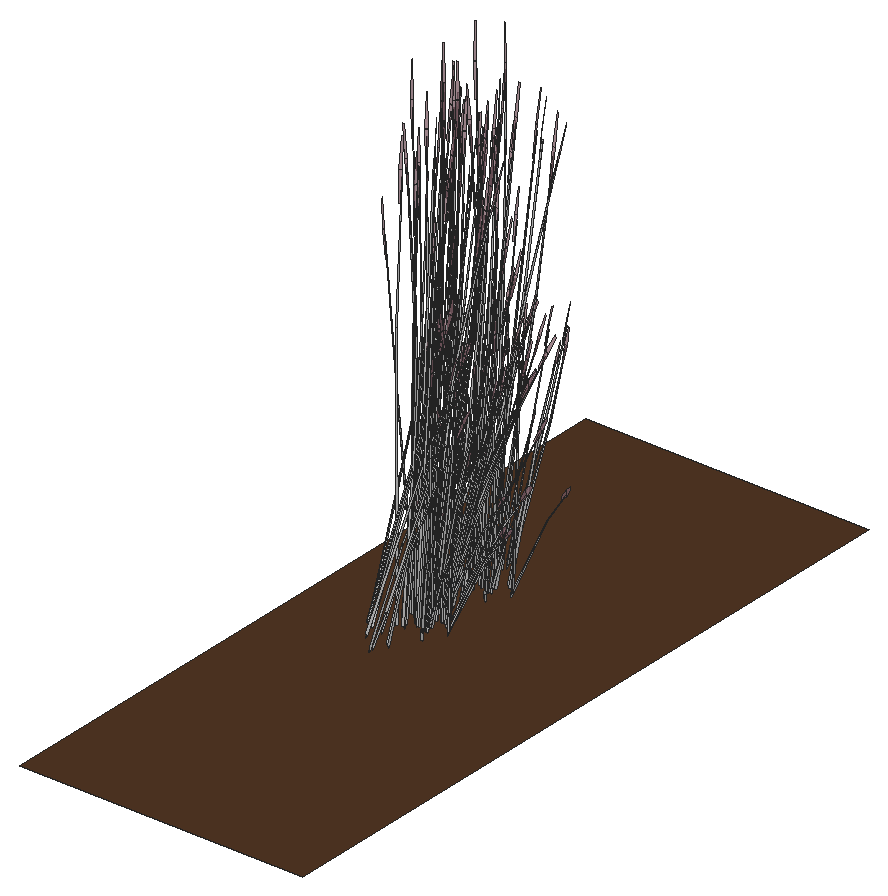
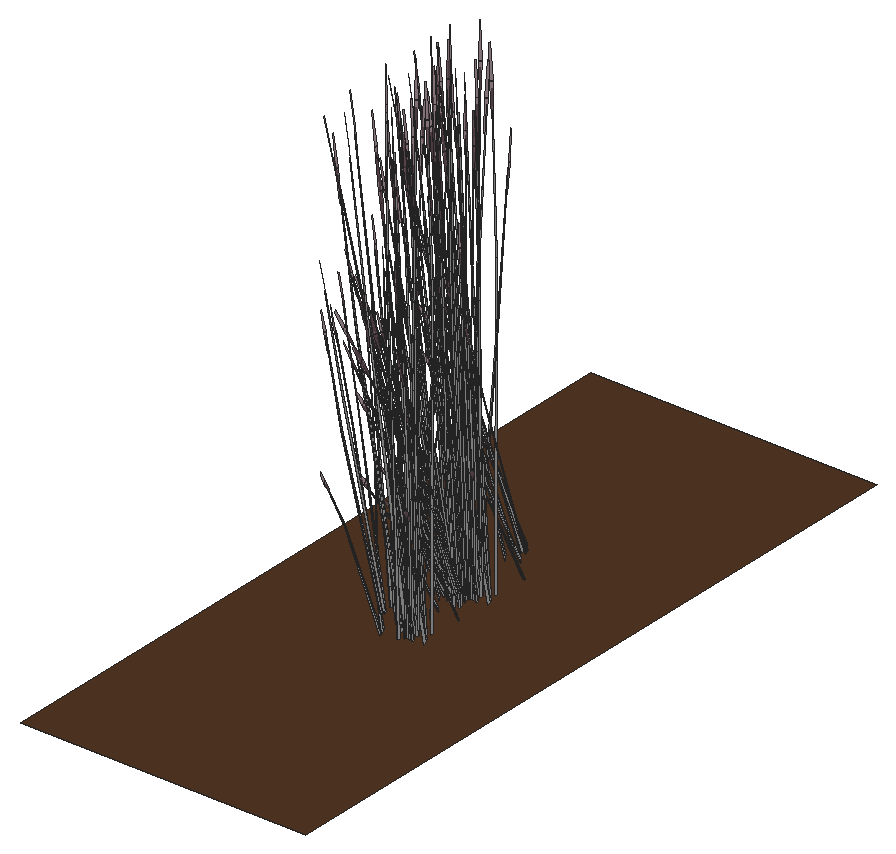
# SketchUp Ruby script. Lengths in inches.
U = 1.inch
M = Sketchup.active_model
def pt(a) = Geom::Point3d.new(a.map { |v| v * U })
def face(e, loops, mat)
  f = e.add_face(loops[0].map { |a| pt(a) })
  loops[1..].each { |l| e.add_face(l.map { |a| pt(a) }).erase! }
  f.material = f.back_material = mat if mat
  f
end
# faces: each face lists its corners as indices into pts; further lists are holes
def faces(e, pts, list, mat = nil) = list.each { |f| face(e, (f[0].is_a?(Array) ? f : [f]).map { |l| l.map { |i| pts[i] } }, mat) }
# xy, xz, yz: faces in a plane at the given z, y or x. An outline is a flat list of corners, or four numbers for a rectangle; further outlines are holes
def ring(l) = l.size == 4 ? [[l[0], l[1]], [l[2], l[1]], [l[2], l[3]], [l[0], l[3]]] : l.each_slice(2).to_a
def flat(e, list, mat, &to3) = list.each { |f| face(e, (f[0].is_a?(Array) ? f : [f]).map { |l| ring(l).map { |u, v| to3.(u, v) } }, mat) }
def xy(e, z, list, mat = nil) = flat(e, list, mat) { |x, y| [x, y, z] }
def xz(e, y, list, mat = nil) = flat(e, list, mat) { |x, z| [x, y, z] }
def yz(e, x, list, mat = nil) = flat(e, list, mat) { |y, z| [x, y, z] }
def lines(e, pts, list) = list.each { |a, b| e.add_line(pt(pts[a]), pt(pts[b])) }
# prism: a flat outline (further loops are holes) pulled along v
def prism(e, loops, v, mat = nil)
  f = face(e, loops, mat); d = Geom::Vector3d.new(v.map { |x| x * U })
  f.pushpull(f.normal.samedirection?(d) ? d.length : -d.length)
end
def box(e, o, s, mat = nil) = prism(e, [[o, [o[0] + s[0], o[1], o[2]], [o[0] + s[0], o[1] + s[1], o[2]], [o[0], o[1] + s[1], o[2]]]], [0, 0, s[2]], mat)
def at(x, y, z, deg = 0) = Geom::Transformation.translation(pt([x, y, z])) * Geom::Transformation.rotation(ORIGIN, Z_AXIS, deg.degrees)
def axes(o, x, y, z) = Geom::Transformation.new([*x, 0, *y, 0, *z, 0, *pt(o).to_a, 1])
def part(name) = M.definitions.add(name)
# library, detail: a bought-in or finely detailed component or shape, given as its bounding box
def library(name, o, s) = part(name).tap { |d| box(d.entities, o, s) }
def detail(e, o, s) = box(e.add_group.entities, o, s)
def put(e, d, t, mat = nil) = e.add_instance(d, t).tap { |i| i.material = mat if mat }
def group(e, t, mat = nil) = e.add_group.tap { |g| g.transformation = t; g.material = mat if mat }.entities
root = M.entities
M.materials.add("LightPink_Translucent").color = [144, 107, 117]
M.materials["LightPink_Translucent"].alpha = 0.75
M.materials.add("Wood_Veneer_15_1K").color = [81, 54, 35]
M.materials.add("[_0053_Ivory_]").color = [200, 200, 200]
c1 = part("blade")
p = [[2.15,0.21,22],[0,0.17,0],[0.09,0.45,0],[2.18,0.31,22],[2.29,0.31,22],[0.38,0.45,0],
  [2.48,0.24,33],[2.49,0.24,33],[2.48,0.22,33]]
faces(c1.entities,p,[[0,1,2,3],[4,5,2,3],[6,3,4,7],[8,0,3,6]])
c2 = part("seeds")
p = [[0.3,-0.1,1.38],[-0.01,-0.03,1.59],[-0.01,-0.03,0.03],[0.14,-0.07,-0.07],[0.29,-0.03,3],[0.15,0.01,3.11]]
faces(c2.entities,p,[[0,1,2,3],[1,0,4,5]],"LightPink_Translucent")
c3 = part("blade with seeds")
put(c3.entities,c1,at(0,0,0))
put(c3.entities,c2,axes([2.4,0.25,30.99],[1.5799,-0.05474,1.17369],[-0.12525,1.92788,0.29478],[-0.07173,-0.02425,1.56792]))
xy(root,252,[[617.51,269.15,653.51,359.15]],"Wood_Veneer_15_1K")
put(root,c3,axes([631.24,314.625,253.86],[0.29468,-0.56664,-0.44739],[0.61229,0.27271,0.21531],[0,-0.13062,1.43643]),"[_0053_Ivory_]")
put(root,c3,axes([631.24,324.73,253.86],[0.29468,-0.56664,-0.44739],[0.61229,0.27271,0.21531],[0,-0.13062,1.43643]),"[_0053_Ivory_]")
put(root,c3,axes([631.99,316.45,253.86],[-0.19817,-0.54216,0],[0.56587,-0.18986,0],[0,0,1.54371]),"[_0053_Ivory_]")
put(root,c3,axes([631.27,307.21,253.15],[0.09829,-0.03422,1.76342],[0.59126,0.18834,-0.26939],[0.01729,0.21228,0.30037]),"[_0053_Ivory_]")
put(root,c3,axes([631.27,317.6,253.15],[0.09829,-0.03422,1.76342],[0.59126,0.18834,-0.26939],[0.01729,0.21228,0.30037]),"[_0053_Ivory_]")
put(root,c3,axes([631.4,307.4,256.18],[-0.1831,0.48359,-0.35414],[-0.53419,-0.14105,0.4572],[0.04898,0.1947,0.87481]),"[_0053_Ivory_]")
put(root,c3,axes([631.4,317.79,256.18],[-0.1831,0.48359,-0.35414],[-0.53419,-0.14105,0.4572],[0.04898,0.1947,0.87481]),"[_0053_Ivory_]")
put(root,c3,axes([632.79,315.38,253.86],[-0.29468,0.56664,-0.44739],[-0.61229,-0.27271,0.21531],[0,0.13062,1.43643]),"[_0053_Ivory_]")
put(root,c3,axes([633.95,315.04,254.13],[-0.47719,-0.45806,0.17642],[0.48088,-0.44429,0.35086],[-0.0527,0.09355,1.60407]),"[_0053_Ivory_]")
put(root,c3,axes([632.31,314.78,253.86],[0,-0.72763,0],[0.75945,0,0],[0,0,1.79456]),"[_0053_Ivory_]")
put(root,c3,axes([632.31,324.88,253.86],[0,-0.72763,0],[0.75945,0,0],[0,0,1.79456]),"[_0053_Ivory_]")
put(root,c3,axes([631.6,314.91,254.09],[0.68433,0.30479,0.24065],[-0.32934,0.63331,0.50002],[0,-0.14599,1.60543]),"[_0053_Ivory_]")
put(root,c3,axes([631.6,325.01,254.09],[0.68433,0.30479,0.24065],[-0.32934,0.63331,0.50002],[0,-0.14599,1.60543]),"[_0053_Ivory_]")
put(root,c3,axes([632.6875,315.07,253.95],[0,0.72727,-0.05637],[-0.75945,0,0],[0,0.02286,1.79368]),"[_0053_Ivory_]")
put(root,c3,axes([631.38,314.48,254.37],[-0.65953,0.03882,0.44739],[-0.05964,-0.64439,-0.21531],[0.11807,-0.06531,1.43643]),"[_0053_Ivory_]")
put(root,c3,axes([631.38,324.59,254.37],[-0.65953,0.03882,0.44739],[-0.05964,-0.64439,-0.21531],[0.11807,-0.06531,1.43643]),"[_0053_Ivory_]")
put(root,c3,axes([631.07,313.375,254.13],[-0.17545,0.62497,0.17642],[-0.64204,-0.17686,0.35086],[0.11091,-0.00304,1.60407]),"[_0053_Ivory_]")
put(root,c3,axes([631.07,323.48,254.13],[-0.17545,0.62497,0.17642],[-0.64204,-0.17686,0.35086],[0.11091,-0.00304,1.60407]),"[_0053_Ivory_]")
put(root,c3,axes([632.32,316.47,253.94],[0.26406,0.72244,-0.06012],[-0.7545,0.25315,0],[0.00922,0.02523,1.72173]),"[_0053_Ivory_]")
put(root,c3,axes([630.76,312.61,254.03],[-0.37973,-0.63014,0],[0.6353,-0.35142,-0.51607],[0.14469,-0.08004,1.63711]),"[_0053_Ivory_]")
put(root,c3,axes([630.76,322.71,254.03],[-0.37973,-0.63014,0],[0.6353,-0.35142,-0.51607],[0.14469,-0.08004,1.63711]),"[_0053_Ivory_]")
put(root,c3,axes([631.46,306.96,256.63],[0.28988,0.51132,-0.71045],[-0.59671,0.28496,0.08574],[0.06778,0.24706,1.00501]),"[_0053_Ivory_]")
put(root,c3,axes([631.46,317.35,256.63],[0.28988,0.51132,-0.71045],[-0.59671,0.28496,0.08574],[0.06778,0.24706,1.00501]),"[_0053_Ivory_]")
put(root,c3,axes([634.51,315.53,253.85],[-0.75908,-0.00503,-0.04976],[0,-0.70283,0.49943],[-0.02386,0.16,1.58352]),"[_0053_Ivory_]")
put(root,c3,axes([633.01,313.41,254.13],[-0.65264,0.16691,0.17642],[-0.16115,-0.62115,0.35086],[0.05821,0.0905,1.60407]),"[_0053_Ivory_]")
put(root,c3,axes([632.35,321.1875,254.42],[0.07791,0.3667,1.1486],[-0.43222,-0.2031,0.84392],[0.04651,-0.18776,0.25299]),"[_0053_Ivory_]")
put(root,c3,axes([631.95,314.32,254.01],[-0.50358,0.57069,0.45755],[-0.59827,-0.50377,0.17955],[0.1214,-0.05695,1.58856]),"[_0053_Ivory_]")
put(root,c3,axes([631.95,324.42,254.01],[-0.50358,0.57069,0.45755],[-0.59827,-0.50377,0.17955],[0.1214,-0.05695,1.58856]),"[_0053_Ivory_]")
put(root,c3,axes([632.81,315.22,253.87],[0.42396,0.40619,0],[-0.42396,0.40619,0],[0,0,1.69266]),"[_0053_Ivory_]")
put(root,c3,axes([632.8,314.74,254.37],[0.29468,-0.56664,0.44739],[0.61229,0.27271,-0.21531],[0,0.13062,1.43643]),"[_0053_Ivory_]")
put(root,c3,axes([632.55,316.71,253.86],[0.61229,0.28233,0],[-0.29468,0.58663,0],[0,0,1.74954]),"[_0053_Ivory_]")
put(root,c3,axes([631.67,307.07,256.33],[0.59704,0.15764,-0.51099],[-0.20464,0.54049,-0.3958],[0.05475,0.21761,0.97773]),"[_0053_Ivory_]")
put(root,c3,axes([631.67,317.46,256.33],[0.59704,0.15764,-0.51099],[-0.20464,0.54049,-0.3958],[0.05475,0.21761,0.97773]),"[_0053_Ivory_]")
put(root,c3,axes([632.6,314.61,254.03],[-0.76764,-0.13249,0.49198],[0.15622,-0.74829,0.19306],[0.11218,0.07226,1.70813]),"[_0053_Ivory_]")
put(root,c3,axes([634.35,315.63,253.68],[-0.42396,0.39235,-0.30978],[-0.42396,-0.39235,0.30978],[0,0.12637,1.38974]),"[_0053_Ivory_]")
put(root,c3,axes([633.14,315.56,253.75],[0.2227,0.57576,-0.69212],[-0.64151,0.20736,-0.18165],[0.02462,0.19497,1.52773]),"[_0053_Ivory_]")
put(root,c3,axes([632.82,314.9375,253.86],[0.67951,0,0],[0,0.65103,0],[0,0,1.78407]),"[_0053_Ivory_]")
put(root,c3,axes([632.82,325.04,253.86],[0.67951,0,0],[0,0.65103,0],[0,0,1.78407]),"[_0053_Ivory_]")
put(root,c3,axes([632.17,314.22,254.37],[-0.36485,-0.52782,0.44739],[0.55265,-0.37168,-0.21531],[0.11807,0.06531,1.43643]),"[_0053_Ivory_]")
put(root,c3,axes([632.17,324.33,254.37],[-0.36485,-0.52782,0.44739],[0.55265,-0.37168,-0.21531],[0.11807,0.06531,1.43643]),"[_0053_Ivory_]")
put(root,c3,axes([631.5,314.35,254.32],[-0.07077,-0.71755,-0.29095],[0.73712,-0.04339,-0.50002],[0.1298,-0.09558,1.59708]),"[_0053_Ivory_]")
put(root,c3,axes([631.5,324.45,254.32],[-0.07077,-0.71755,-0.29095],[0.73712,-0.04339,-0.50002],[0.1298,-0.09558,1.59708]),"[_0053_Ivory_]")
put(root,c3,axes([633.06,314.87,254.27],[0.56587,-0.18339,0.1448],[0.19817,0.52368,-0.41347],[0,0.11525,1.26744]),"[_0053_Ivory_]")
put(root,c3,axes([633.27,322.95,256.33],[-0.43478,-0.42253,-0.51099],[0.45929,-0.37004,-0.3958],[0.06615,-0.21468,0.97773]),"[_0053_Ivory_]")
put(root,c3,axes([632.86,314.91,254.32],[0.68399,0.30005,-0.29095],[-0.32934,0.63331,-0.50002],[0.0215,0.15549,1.59708]),"[_0053_Ivory_]")
put(root,c3,axes([631.41,312.76,253.68],[0.56663,0.1556,-0.30978],[-0.14267,0.54795,0.30978],[0.11423,-0.06319,1.38974]),"[_0053_Ivory_]")
put(root,c3,axes([631.41,322.86,253.68],[0.56663,0.1556,-0.30978],[-0.14267,0.54795,0.30978],[0.11423,-0.06319,1.38974]),"[_0053_Ivory_]")
put(root,c3,axes([632.98,322.2,254.24],[-0.17264,0.12729,1.43002],[-0.51703,-0.22279,-0.30754],[0.09584,-0.27707,0.61141]),"[_0053_Ivory_]")
put(root,c3,axes([634.35,315.06,254.13],[0,-0.62885,0.49651],[0.67951,0,0],[0,0.14322,1.57504]),"[_0053_Ivory_]")
put(root,c3,axes([634.64,315.64,253.67],[0,0.62885,-0.49651],[-0.67951,0,0],[0,0.14322,1.57504]),"[_0053_Ivory_]")
put(root,c3,axes([631.27,312.51,253.67],[0.56842,-0.31443,-0.49651],[0.33976,0.56381,0],[0.12946,-0.07161,1.57504]),"[_0053_Ivory_]")
put(root,c3,axes([631.27,322.61,253.67],[0.56842,-0.31443,-0.49651],[0.33976,0.56381,0],[0.12946,-0.07161,1.57504]),"[_0053_Ivory_]")
put(root,c3,axes([632.01,305.95,255.53],[-0.13883,-0.2019,1.71376],[0.64153,-0.16998,0.13857],[0.14499,0.31697,0.73262]),"[_0053_Ivory_]")
put(root,c3,axes([632.01,316.34,255.53],[-0.13883,-0.2019,1.71376],[0.64153,-0.16998,0.13857],[0.14499,0.31697,0.73262]),"[_0053_Ivory_]")
put(root,c3,axes([632.41,314.07,254.27],[0.11717,-0.56122,0.1448],[0.57245,0.09742,-0.41347],[0.10418,0.05763,1.26744]),"[_0053_Ivory_]")
put(root,c3,axes([632.41,324.18,254.27],[0.11717,-0.56122,0.1448],[0.57245,0.09742,-0.41347],[0.10418,0.05763,1.26744]),"[_0053_Ivory_]")
put(root,c3,axes([633.23,313.09,254.13],[-0.56842,-0.31443,0.49651],[0.33976,-0.56381,0],[0.12946,0.07161,1.57504]),"[_0053_Ivory_]")
put(root,c3,axes([633.23,323.2,254.13],[-0.56842,-0.31443,0.49651],[0.33976,-0.56381,0],[0.12946,0.07161,1.57504]),"[_0053_Ivory_]")
put(root,c3,axes([633.4,323.15,256.63],[0.0158,-0.58168,-0.71045],[0.66548,0.03907,0.08574],[0.07023,-0.24643,1.00501]),"[_0053_Ivory_]")
put(root,c3,axes([632.73,316.38,253.84],[0.63764,-0.21337,-0.19198],[0.22406,0.61462,0.00008],[0.07038,-0.02358,1.73897]),"[_0053_Ivory_]")
put(root,c3,axes([632.74,314.55,253.86],[0.36485,0.52782,-0.44739],[-0.55265,0.37168,0.21531],[0.11807,0.06531,1.43643]),"[_0053_Ivory_]")
put(root,c3,axes([633.68,322.8,256.18],[0.41095,-0.33109,-0.35414],[0.38901,0.37805,0.4572],[0.05919,-0.19208,0.87481]),"[_0053_Ivory_]")
put(root,c3,axes([633.78,316.95,254.42],[-0.34197,-0.18082,1.1486],[0.44156,-0.18372,0.84392],[0.1191,0.15563,0.25299]),"[_0053_Ivory_]")
put(root,c3,axes([632.56,306.36,254.24],[0.01072,-0.20846,1.43002],[0.51218,-0.23285,-0.30754],[0.15811,0.2495,0.61141]),"[_0053_Ivory_]")
put(root,c3,axes([632.56,316.75,254.24],[0.01072,-0.20846,1.43002],[0.51218,-0.23285,-0.30754],[0.15811,0.2495,0.61141]),"[_0053_Ivory_]")
put(root,c3,axes([631.95,313.8,253.71],[0.40909,-0.47266,-0.62353],[0.50819,0.4286,-0.16365],[0.16393,-0.11791,1.37633]),"[_0053_Ivory_]")
put(root,c3,axes([631.95,323.9,253.71],[0.40909,-0.47266,-0.62353],[0.50819,0.4286,-0.16365],[0.16393,-0.11791,1.37633]),"[_0053_Ivory_]")
put(root,c3,axes([633.74,313.38,253.68],[0.14267,0.54795,-0.30978],[-0.56663,0.1556,0.30978],[0.11423,0.06319,1.38974]),"[_0053_Ivory_]")
put(root,c3,axes([634.81,315.16,254.03],[0.75945,0,0],[0,0.70283,-0.51607],[0,0.16007,1.63711]),"[_0053_Ivory_]")
put(root,c3,axes([632.35,314.25,254.32],[0.61322,-0.4175,-0.29095],[0.40778,0.58992,-0.50002],[0.1513,0.05991,1.59708]),"[_0053_Ivory_]")
put(root,c3,axes([632.35,324.36,254.32],[0.61322,-0.4175,-0.29095],[0.40778,0.58992,-0.50002],[0.1513,0.05991,1.59708]),"[_0053_Ivory_]")
put(root,c3,axes([633.83,307.38,254.32],[-0.38947,-0.01972,1.0506],[0.25721,-0.41888,0.58006],[0.15386,0.14882,0.8241]),"[_0053_Ivory_]")
put(root,c3,axes([633.83,317.77,254.32],[-0.38947,-0.01972,1.0506],[0.25721,-0.41888,0.58006],[0.15386,0.14882,0.8241]),"[_0053_Ivory_]")
put(root,c3,axes([632.65,322.85,255.53],[-0.11309,0.21615,1.71376],[-0.47441,-0.44731,0.13857],[0.21402,-0.27879,0.73262]),"[_0053_Ivory_]")
put(root,c3,axes([630.81,313.88,253.25],[-0.59782,0.25177,1.28929],[-0.19028,-0.72239,0.50096],[0.36709,0.01202,1.46642]),"[_0053_Ivory_]")
put(root,c3,axes([630.81,323.99,253.25],[-0.59782,0.25177,1.28929],[-0.19028,-0.72239,0.50096],[0.36709,0.01202,1.46642]),"[_0053_Ivory_]")
put(root,c3,axes([633,306.8,256.33],[0.59932,-0.14948,-0.51099],[0.10484,0.56611,-0.3958],[0.16097,0.16223,0.97773]),"[_0053_Ivory_]")
put(root,c3,axes([633,317.19,256.33],[0.59932,-0.14948,-0.51099],[0.10484,0.56611,-0.3958],[0.16097,0.16223,0.97773]),"[_0053_Ivory_]")
put(root,c3,axes([633.55,312.76,254.03],[0.37973,-0.63014,0],[0.6353,0.35142,-0.51607],[0.14469,0.08004,1.63711]),"[_0053_Ivory_]")
put(root,c3,axes([633.55,322.87,254.03],[0.37973,-0.63014,0],[0.6353,0.35142,-0.51607],[0.14469,0.08004,1.63711]),"[_0053_Ivory_]")
put(root,c3,axes([634.19,312.49,253.15],[-0.0909,-0.04954,1.76342],[-0.2335,-0.55347,-0.26939],[0.15752,-0.1502,0.30037]),"[_0053_Ivory_]")
put(root,c3,axes([634.19,322.6,253.15],[-0.0909,-0.04954,1.76342],[-0.2335,-0.55347,-0.26939],[0.15752,-0.1502,0.30037]),"[_0053_Ivory_]")
put(root,c3,axes([633.9,313.14,253.67],[0.56842,0.31443,-0.49651],[-0.33976,0.56381,0],[0.12946,0.07161,1.57504]),"[_0053_Ivory_]")
put(root,c3,axes([633.9,323.25,253.67],[0.56842,0.31443,-0.49651],[-0.33976,0.56381,0],[0.12946,0.07161,1.57504]),"[_0053_Ivory_]")
put(root,c3,axes([633.87,317.62,253.15],[0.04425,-0.09079,1.76342],[0.55709,-0.26738,-0.26939],[0.16889,0.13839,0.30037]),"[_0053_Ivory_]")
put(root,c3,axes([634.17,313.82,256.33],[-0.15602,-0.5742,-0.51099],[0.59087,-0.10045,-0.3958],[0.16933,-0.15423,0.97773]),"[_0053_Ivory_]")
put(root,c3,axes([634.17,323.92,256.33],[-0.15602,-0.5742,-0.51099],[0.59087,-0.10045,-0.3958],[0.16933,-0.15423,0.97773]),"[_0053_Ivory_]")
put(root,c3,axes([635.21,316.78,255.58],[-0.11624,-0.52862,-0.03492],[0.54943,-0.12153,-0.15832],[0.11473,0.03351,0.52218]),"[_0053_Ivory_]")
put(root,c3,axes([633.07,314.35,253.71],[0.63179,0.1031,-0.62353],[-0.13332,0.63596,-0.16365],[0.18854,0.07706,1.37633]),"[_0053_Ivory_]")
put(root,c3,axes([635.76,314.72,253.91],[-0.37654,-0.40212,-0.06488],[0.4124,-0.36845,-0.29416],[0.11685,-0.02594,0.97024]),"[_0053_Ivory_]")
put(root,c3,axes([635.76,324.83,253.91],[-0.37654,-0.40212,-0.06488],[0.4124,-0.36845,-0.29416],[0.11685,-0.02594,0.97024]),"[_0053_Ivory_]")
put(root,c3,axes([634.9,312.68,254.42],[-0.2023,0.32011,1.1486],[-0.17388,-0.43009,0.84392],[0.16708,-0.10777,0.25299]),"[_0053_Ivory_]")
put(root,c3,axes([634.9,322.78,254.42],[-0.2023,0.32011,1.1486],[-0.17388,-0.43009,0.84392],[0.16708,-0.10777,0.25299]),"[_0053_Ivory_]")
put(root,c3,axes([632.94,315.71,255.53],[-0.2256,-0.10835,1.71376],[0.46687,-0.45453,0.13857],[0.29098,0.20505,0.73262]),"[_0053_Ivory_]")
put(root,c3,axes([634.61,313.88,256.18],[0.52868,-0.08987,-0.35414],[0.1396,0.51376,0.4572],[0.1515,-0.13799,0.87481]),"[_0053_Ivory_]")
put(root,c3,axes([634.61,323.98,256.18],[0.52868,-0.08987,-0.35414],[0.1396,0.51376,0.4572],[0.1515,-0.13799,0.87481]),"[_0053_Ivory_]")
put(root,c3,axes([634.1875,314.05,256.63],[0.31725,-0.49618,-0.71045],[0.55593,0.35263,0.08574],[0.18942,-0.17977,1.00501]),"[_0053_Ivory_]")
put(root,c3,axes([634.1875,324.16,256.63],[0.31725,-0.49618,-0.71045],[0.55593,0.35263,0.08574],[0.18942,-0.17977,1.00501]),"[_0053_Ivory_]")
put(root,c3,axes([634.18,316.72,256.18],[0.34557,0.39372,-0.35414],[-0.39459,0.37271,0.4572],[0.20048,0.05671,0.87481]),"[_0053_Ivory_]")
put(root,c3,axes([634.45,315.09,256.33],[0.16454,-0.57202,-0.51099],[0.56413,0.19607,-0.3958],[0.22713,-0.05245,0.97773]),"[_0053_Ivory_]")
put(root,c3,axes([634.45,325.2,256.33],[0.16454,-0.57202,-0.51099],[0.56413,0.19607,-0.3958],[0.22713,-0.05245,0.97773]),"[_0053_Ivory_]")
put(root,c3,axes([635.86,315.46,254.42],[-0.37526,0.10382,1.1486],[0.17664,-0.42906,0.84392],[0.19907,0.02936,0.25299]),"[_0053_Ivory_]")
put(root,c3,axes([634.65,313.59,254.24],[-0.21697,-0.01863,1.43002],[-0.22228,-0.49966,-0.30754],[0.26655,-0.14135,0.61141]),"[_0053_Ivory_]")
put(root,c3,axes([634.65,323.7,254.24],[-0.21697,-0.01863,1.43002],[-0.22228,-0.49966,-0.30754],[0.26655,-0.14135,0.61141]),"[_0053_Ivory_]")
put(root,c3,axes([634.79,315.35,256.18],[0.50475,0.17543,-0.35414],[-0.14722,0.5118,0.4572],[0.20322,-0.04693,0.87481]),"[_0053_Ivory_]")
put(root,c3,axes([634.79,325.46,256.18],[0.50475,0.17543,-0.35414],[-0.14722,0.5118,0.4572],[0.20322,-0.04693,0.87481]),"[_0053_Ivory_]")
put(root,c3,axes([633.82,316.46,256.63],[0.60713,0.01514,-0.71045],[-0.04078,0.63759,0.08574],[0.25721,0.06729,1.00501]),"[_0053_Ivory_]")
put(root,c3,axes([635.05,315.26,253.64],[-0.39118,0.07547,1.41583],[-0.06226,-0.6007,0.08104],[0.27398,-0.09092,0.80566]),"[_0053_Ivory_]")
put(root,c3,axes([635.05,325.36,253.64],[-0.39118,0.07547,1.41583],[-0.06226,-0.6007,0.08104],[0.27398,-0.09092,0.80566]),"[_0053_Ivory_]")
put(root,c3,axes([635.48,314.86,253.15],[-0.03174,-0.09547,1.76342],[0.22015,-0.55846,-0.26939],[0.22208,-0.00803,0.30037]),"[_0053_Ivory_]")
put(root,c3,axes([635.48,324.97,253.15],[-0.03174,-0.09547,1.76342],[0.22015,-0.55846,-0.26939],[0.22208,-0.00803,0.30037]),"[_0053_Ivory_]")
put(root,c3,axes([633.42,314.72,255.53],[-0.25192,0.01424,1.71376],[0.16712,-0.61729,0.13857],[0.35901,0.03818,0.73262]),"[_0053_Ivory_]")
put(root,c3,axes([634.34,315.3,256.63],[0.53369,-0.27773,-0.71045],[0.29743,0.5717,0.08574],[0.25786,-0.06494,1.00501]),"[_0053_Ivory_]")
put(root,c3,axes([634.34,325.41,256.63],[0.53369,-0.27773,-0.71045],[0.29743,0.5717,0.08574],[0.25786,-0.06494,1.00501]),"[_0053_Ivory_]")
put(root,c3,axes([635.16,316.15,254.24],[-0.14627,-0.15466,1.43002],[0.19032,-0.51164,-0.30754],[0.29594,0.06931,0.61141]),"[_0053_Ivory_]")
